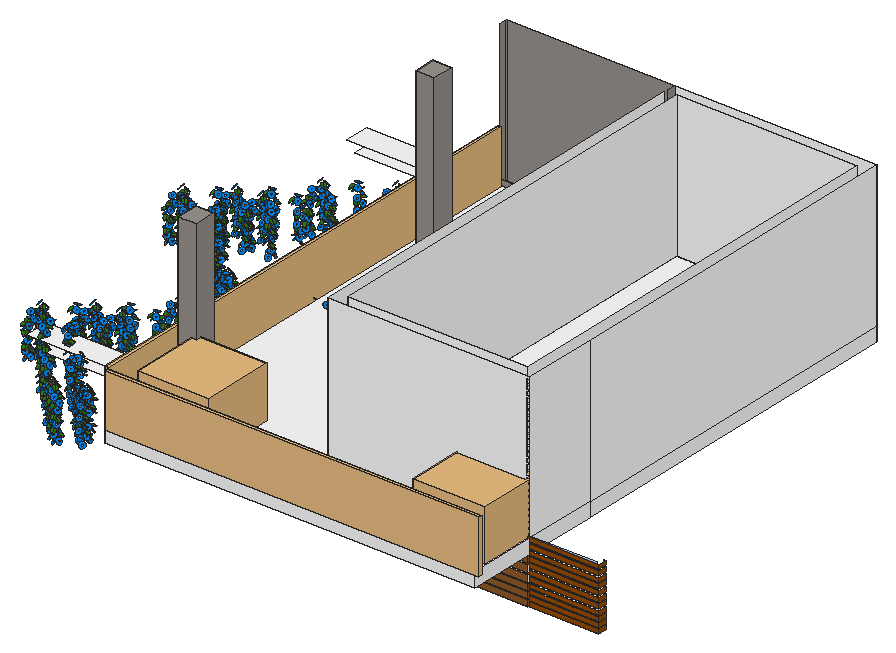
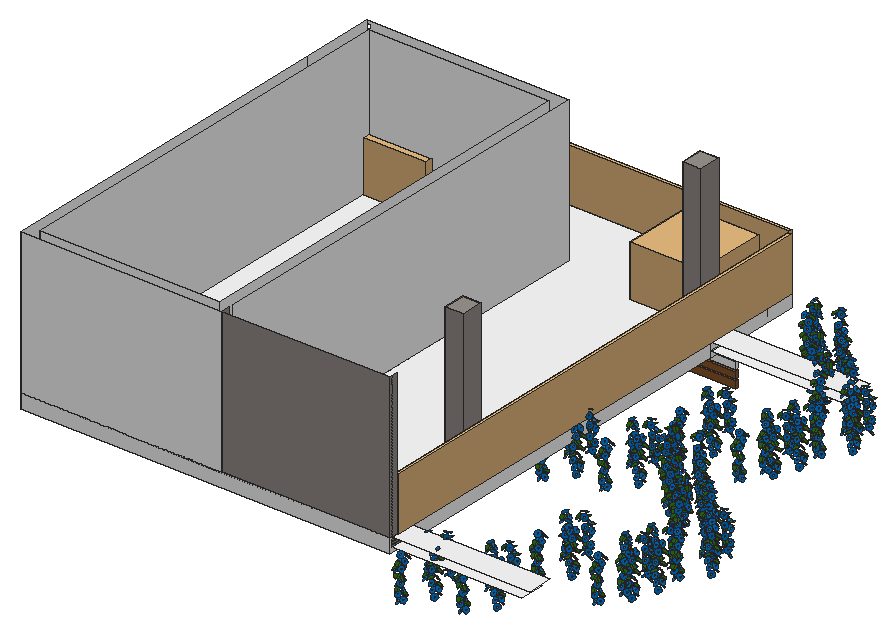
# SketchUp Ruby script. Lengths in inches.
U = 1.inch
M = Sketchup.active_model
def pt(a) = Geom::Point3d.new(a.map { |v| v * U })
def face(e, loops, mat)
  f = e.add_face(loops[0].map { |a| pt(a) })
  loops[1..].each { |l| e.add_face(l.map { |a| pt(a) }).erase! }
  f.material = f.back_material = mat if mat
  f
end
# faces: each face lists its corners as indices into pts; further lists are holes
def faces(e, pts, list, mat = nil) = list.each { |f| face(e, (f[0].is_a?(Array) ? f : [f]).map { |l| l.map { |i| pts[i] } }, mat) }
# xy, xz, yz: faces in a plane at the given z, y or x. An outline is a flat list of corners, or four numbers for a rectangle; further outlines are holes
def ring(l) = l.size == 4 ? [[l[0], l[1]], [l[2], l[1]], [l[2], l[3]], [l[0], l[3]]] : l.each_slice(2).to_a
def flat(e, list, mat, &to3) = list.each { |f| face(e, (f[0].is_a?(Array) ? f : [f]).map { |l| ring(l).map { |u, v| to3.(u, v) } }, mat) }
def xy(e, z, list, mat = nil) = flat(e, list, mat) { |x, y| [x, y, z] }
def xz(e, y, list, mat = nil) = flat(e, list, mat) { |x, z| [x, y, z] }
def yz(e, x, list, mat = nil) = flat(e, list, mat) { |y, z| [x, y, z] }
def lines(e, pts, list) = list.each { |a, b| e.add_line(pt(pts[a]), pt(pts[b])) }
# prism: a flat outline (further loops are holes) pulled along v
def prism(e, loops, v, mat = nil)
  f = face(e, loops, mat); d = Geom::Vector3d.new(v.map { |x| x * U })
  f.pushpull(f.normal.samedirection?(d) ? d.length : -d.length)
end
def box(e, o, s, mat = nil) = prism(e, [[o, [o[0] + s[0], o[1], o[2]], [o[0] + s[0], o[1] + s[1], o[2]], [o[0], o[1] + s[1], o[2]]]], [0, 0, s[2]], mat)
def at(x, y, z, deg = 0) = Geom::Transformation.translation(pt([x, y, z])) * Geom::Transformation.rotation(ORIGIN, Z_AXIS, deg.degrees)
def axes(o, x, y, z) = Geom::Transformation.new([*x, 0, *y, 0, *z, 0, *pt(o).to_a, 1])
def part(name) = M.definitions.add(name)
# library, detail: a bought-in or finely detailed component or shape, given as its bounding box
def library(name, o, s) = part(name).tap { |d| box(d.entities, o, s) }
def detail(e, o, s) = box(e.add_group.entities, o, s)
def put(e, d, t, mat = nil) = e.add_instance(d, t).tap { |i| i.material = mat if mat }
def group(e, t, mat = nil) = e.add_group.tap { |g| g.transformation = t; g.material = mat if mat }.entities
root = M.entities
M.materials.add("[Color C07]").color = [153, 76, 0]
M.materials.add("[Color M00]").color = [255, 255, 255]
M.materials.add("[Granite Tile]").color = [155, 148, 143]
M.materials.add("[Translucent Glass Blue]").color = [100, 149, 237]
M.materials["[Translucent Glass Blue]"].alpha = 0.5
M.materials.add("[Wood Floor Parquet]").color = [145, 89, 39]
M.materials.add("skp avat flo 1").color = [0, 129, 229]
M.materials.add("skp avat flo 2").color = [47, 120, 22]
c1 = part("Gruppe\#2")
xy(c1.entities,0,[[6.69,0,4.96,0.23,3.03,1.59,1.96,1.96,0.9,3.35,0.9,5.71,0,6.69,0.23,8.43,1.96,10,3.35,12.49,4.67,13.04,7.04,12.49,8.72,13.04,10.04,12.49,11.43,11.43,12.05,9.15,13.39,6.69,13.16,4.96,12.49,3.35,10.41,2.22,8.43,0.23]],"skp avat flo 1")
c2 = part("Gruppe\#12")
xy(c2.entities,0,[[1.18,0.5,1.36,0.52,1.52,0.59,1.67,0.7,1.77,0.84,1.84,1,1.87,1.18,1.84,1.36,1.77,1.52,1.67,1.67,1.52,1.77,1.36,1.84,1.18,1.87,1,1.84,0.84,1.77,0.7,1.67,0.59,1.52,0.52,1.36,0.5,1.18,0.52,1,0.59,0.84,0.7,0.7,0.84,0.59,1,0.52]])
c3 = part("f.st. wop plant 01 blüte")
put(c3.entities,c1,at(0,0,0))
put(c3.entities,c2,at(5.65,5.41,0.39))
c4 = part("Gruppe\#5")
xy(c4.entities,0.96,[[13.97,0.22,8.73,4.42,7.37,10.11,8.43,14.53,13.97,16.39]],"skp avat flo 2")
p = [[13.97,0.22,0.96],[13.97,16.39,0.96],[17.89,14.53,4.875],[18.64,10.11,5.625],[17.67,4.42,4.66]]
faces(c4.entities,p,[[0,1,2,3,4]],"skp avat flo 2")
c5 = part("f.st. wop plant 01 blatt")
put(c5.entities,c4,axes([0.99,0,4.74],[0.91566,0,-0.40195],[0,1,0],[0.40195,0,0.91566]))
c6 = part("Gruppe\#10")
put(c6.entities,c3,axes([4.61,0.45,57.14],[0.99373,-0.06775,-0.08889],[0.11172,0.62588,0.77188],[0.00335,-0.77697,0.62953]))
put(c6.entities,c3,axes([12.4,0.4,0.59],[0.70061,0.70799,-0.08889],[-0.40079,0.49353,0.77188],[0.59035,-0.50516,0.62953]))
put(c6.entities,c3,axes([24.4375,6.09,17.58],[-0.05734,0.99439,-0.08889],[-0.63495,0.03239,0.77188],[0.77043,0.1007,0.62953]))
put(c6.entities,c3,axes([1.11,8.09,13.25],[0.88983,-0.44754,-0.08889],[0.34553,0.53368,0.77188],[-0.298,-0.71756,0.62953]))
put(c6.entities,c3,axes([23.26,15,37.53],[-0.84836,0.52191,-0.08889],[-0.38985,-0.50222,0.77188],[0.35821,0.68948,0.62953]))
put(c6.entities,c3,axes([12.67,23.61,24.88],[-0.75852,-0.64555,-0.08889],[0.35717,-0.52596,0.77188],[-0.54504,0.55374,0.62953]))
put(c6.entities,c3,axes([20.43,22.9,81.42],[-0.98432,0.15238,-0.08889],[-0.16477,-0.61405,0.77188],[0.06303,0.77442,0.62953]))
put(c6.entities,c3,axes([1.76,2.9,29.21],[0.93833,-0.33412,-0.08889],[0.27691,0.5723,0.77188],[-0.20703,-0.74889,0.62953]))
put(c6.entities,c3,axes([13.59,0.5,77.09],[0.62412,0.77625,-0.08889],[-0.4494,0.44972,0.77188],[0.63915,-0.4418,0.62953]))
put(c6.entities,c3,axes([-1.26,15.51,69.79],[0.24265,-0.96603,-0.08889],[0.62977,0.08716,0.77188],[-0.73791,-0.24328,0.62953]))
put(c6.entities,c3,axes([22.04,17.92,65.46],[-0.95793,0.27287,-0.08889],[-0.2394,-0.58898,0.77188],[0.15827,0.76069,0.62953]))
put(c6.entities,c3,axes([9.51,23.35,52.81],[-0.55554,-0.82673,-0.08889],[0.48617,-0.40969,0.77188],[-0.67455,0.38559,0.62953]))
put(c6.entities,c3,axes([0.1875,18.97,41.86],[-0.02781,-0.99565,-0.08889],[0.62986,-0.08651,0.77188],[-0.77621,-0.03452,0.62953]))
put(c6.entities,c3,axes([24.98,7.4,94.08],[-0.15925,0.98323,-0.08889],[-0.63491,-0.03305,0.77188],[0.75599,0.17936,0.62953]))
put(c6.entities,c3,axes([21.5,21.98,4.93],[-0.96344,0.25275,-0.08889],[-0.22702,-0.59386,0.77188],[0.1423,0.76384,0.62953]))
put(c6.entities,c3,axes([1.57,6.98,89.75],[0.93112,-0.3537,-0.08889],[0.28884,0.56637,0.77188],[-0.22267,-0.74439,0.62953]))
put(c6.entities,c5,axes([9.37,32.32,90.95],[-0.51317,-0.65235,0],[0.5996,-0.47167,0.32697],[-0.25699,0.20216,0.76288]))
put(c6.entities,c5,axes([33.81,6.72,78.35],[-0.27992,0.78137,0],[-0.71819,-0.25729,0.32697],[0.30782,0.11027,0.76288]))
put(c6.entities,c5,axes([-9.46,14.86,61.47],[0.53029,-0.63851,0],[0.58688,0.4874,0.32697],[-0.25154,-0.2089,0.76288]))
put(c6.entities,c5,axes([21.49,-6.15,66.98],[0.2591,0.78852,0],[-0.72476,0.23815,0.32697],[0.31063,-0.10207,0.76288]))
put(c6.entities,c5,axes([32.03,5.27,54.38],[-0.36397,0.74594,0],[-0.68562,-0.33454,0.32697],[0.29386,0.14338,0.76288]))
put(c6.entities,c5,axes([30.63,20.6,49.31],[-0.77544,0.29596,0],[-0.27203,-0.71273,0.32697],[0.11659,0.30548,0.76288]))
put(c6.entities,c5,axes([32.03,5.27,27.16],[-0.36397,0.74594,0],[-0.68562,-0.33454,0.32697],[0.29386,0.14338,0.76288]))
put(c6.entities,c5,axes([17.4375,27.53,13.8125],[-0.76735,-0.23527,0.21148],[0.29408,-0.735,0.24937],[0.11659,0.30548,0.76288]))
put(c6.entities,c5,axes([-9.46,14.86,34.24],[0.53029,-0.63851,0],[0.58688,0.4874,0.32697],[-0.25154,-0.2089,0.76288]))
c7 = part("Gruppe\#9")
put(c7.entities,c3,axes([2.2,1.62,57.61],[0.97169,-0.0623,-0.22792],[0.22172,0.57378,0.78843],[0.08166,-0.81664,0.57134]))
put(c7.entities,c3,axes([-1.48,7.53,1.27],[0.68093,0.71536,-0.15682],[-0.22028,0.40428,0.88771],[0.69843,-0.56993,0.43287]))
put(c7.entities,c3,axes([13.97,11.34,15.86],[-0.0542,0.99797,0.03349],[-0.45869,-0.05467,0.88691],[0.88694,0.03271,0.46072]))
put(c7.entities,c3,axes([-9.71,13.74,16.77],[0.84218,-0.4326,-0.32186],[0.5102,0.4462,0.73526],[-0.17446,-0.78343,0.59649]))
put(c7.entities,c3,axes([17.17,17.99,36.46],[-0.83727,0.52624,0.14846],[-0.23006,-0.58536,0.77745],[0.49603,0.61679,0.61117]))
put(c7.entities,c3,axes([4.35,27.92,27.32],[-0.77345,-0.63385,0.00301],[0.4998,-0.60694,0.61792],[-0.38984,0.47943,0.78623]))
put(c7.entities,c3,axes([20.43,22.9,81.42],[-0.98432,0.15238,-0.08889],[-0.16477,-0.61405,0.77188],[0.06303,0.77442,0.62953]))
put(c7.entities,c3,axes([-5.84,6.82,31.58],[0.89192,-0.31974,-0.31975],[0.44391,0.4844,0.75386],[-0.08616,-0.81432,0.57398]))
put(c7.entities,c3,axes([13.59,0.5,77.09],[0.62412,0.77625,-0.08889],[-0.4494,0.44972,0.77188],[0.63915,-0.4418,0.62953]))
put(c7.entities,c3,axes([-1.26,15.51,69.79],[0.24265,-0.96603,-0.08889],[0.62977,0.08716,0.77188],[-0.73791,-0.24328,0.62953]))
put(c7.entities,c3,axes([20.77,18.5,64.59],[-0.95848,0.27864,0.06062],[-0.13765,-0.63827,0.75741],[0.24973,0.71762,0.65012]))
put(c7.entities,c3,axes([6.6875,24.75,54.15],[-0.57029,-0.8188,-0.06577],[0.58283,-0.45976,0.67002],[-0.57885,0.34377,0.73942]))
put(c7.entities,c3,axes([-4.08,21.11,44.3125],[-0.04911,-0.98765,-0.14878],[0.72825,-0.13735,0.67141],[-0.68355,-0.07538,0.726]))
put(c7.entities,c3,axes([24.98,7.4,94.08],[-0.15925,0.98323,-0.08889],[-0.63491,-0.03305,0.77188],[0.75599,0.17936,0.62953]))
put(c7.entities,c3,axes([8.77,28.52,5.9],[-0.95532,0.25842,0.14346],[-0.07274,-0.676,0.7333],[0.28648,0.6901,0.6646]))
put(c7.entities,c3,axes([1.57,6.98,89.75],[0.93112,-0.3537,-0.08889],[0.28884,0.56637,0.77188],[-0.22267,-0.74439,0.62953]))
put(c7.entities,c5,axes([9.37,32.32,90.95],[-0.51317,-0.65235,0],[0.5996,-0.47167,0.32697],[-0.25699,0.20216,0.76288]))
put(c7.entities,c5,axes([33.81,6.72,78.35],[-0.27992,0.78137,0],[-0.71819,-0.25729,0.32697],[0.30782,0.11027,0.76288]))
put(c7.entities,c5,axes([-11.01,15.72,64.74],[0.51926,-0.63742,-0.11388],[0.63054,0.46456,0.27478],[-0.14729,-0.25842,0.77487]))
put(c7.entities,c5,axes([20.21,-5.625,64.6],[0.26417,0.78668,0.01588],[-0.67119,0.21655,0.43762],[0.41063,-0.15212,0.70508]))
put(c7.entities,c5,axes([29.04,6.59,51.45],[-0.35348,0.74452,0.09816],[-0.63785,-0.35493,0.39506],[0.39635,0.09281,0.72332]))
put(c7.entities,c5,axes([27.11,22.23,47.625],[-0.76537,0.29574,0.12508],[-0.23173,-0.73252,0.31403],[0.22228,0.25465,0.75805]))
put(c7.entities,c5,axes([23.375,9.49,23.48],[-0.34051,0.7404,0.15735],[-0.60881,-0.37042,0.42548],[0.44978,0.05914,0.69506]))
put(c7.entities,c5,axes([6.77,33.04,15.99],[-0.71083,-0.25923,0.3412],[0.32455,-0.75723,0.10082],[0.2798,0.21977,0.74988]))
put(c7.entities,c5,axes([-15.51,18.125,40.12],[0.50532,-0.63318,-0.18065],[0.65217,0.44994,0.24724],[-0.09068,-0.29247,0.77145]))
c8 = part("Gruppe\#11")
put(c8.entities,c3,axes([4.61,0.45,57.14],[0.99373,-0.06775,-0.08889],[0.11172,0.62588,0.77188],[0.00335,-0.77697,0.62953]))
put(c8.entities,c3,axes([12.4,0.4,0.59],[0.70061,0.70799,-0.08889],[-0.40079,0.49353,0.77188],[0.59035,-0.50516,0.62953]))
put(c8.entities,c3,axes([24.4375,6.09,17.58],[-0.05734,0.99439,-0.08889],[-0.63495,0.03239,0.77188],[0.77043,0.1007,0.62953]))
put(c8.entities,c3,axes([1.11,8.09,13.25],[0.88983,-0.44754,-0.08889],[0.34553,0.53368,0.77188],[-0.298,-0.71756,0.62953]))
put(c8.entities,c3,axes([23.26,15,37.53],[-0.84836,0.52191,-0.08889],[-0.38985,-0.50222,0.77188],[0.35821,0.68948,0.62953]))
put(c8.entities,c3,axes([12.67,23.61,24.88],[-0.75852,-0.64555,-0.08889],[0.35717,-0.52596,0.77188],[-0.54504,0.55374,0.62953]))
put(c8.entities,c3,axes([20.43,22.9,81.42],[-0.98432,0.15238,-0.08889],[-0.16477,-0.61405,0.77188],[0.06303,0.77442,0.62953]))
put(c8.entities,c3,axes([1.76,2.9,29.21],[0.93833,-0.33412,-0.08889],[0.27691,0.5723,0.77188],[-0.20703,-0.74889,0.62953]))
put(c8.entities,c3,axes([13.59,0.5,77.09],[0.62412,0.77625,-0.08889],[-0.4494,0.44972,0.77188],[0.63915,-0.4418,0.62953]))
put(c8.entities,c3,axes([-1.26,15.51,69.79],[0.24265,-0.96603,-0.08889],[0.62977,0.08716,0.77188],[-0.73791,-0.24328,0.62953]))
put(c8.entities,c3,axes([22.04,17.92,65.46],[-0.95793,0.27287,-0.08889],[-0.2394,-0.58898,0.77188],[0.15827,0.76069,0.62953]))
put(c8.entities,c3,axes([9.51,23.35,52.81],[-0.55554,-0.82673,-0.08889],[0.48617,-0.40969,0.77188],[-0.67455,0.38559,0.62953]))
put(c8.entities,c3,axes([0.1875,18.97,41.86],[-0.02781,-0.99565,-0.08889],[0.62986,-0.08651,0.77188],[-0.77621,-0.03452,0.62953]))
put(c8.entities,c3,axes([24.98,7.4,94.08],[-0.15925,0.98323,-0.08889],[-0.63491,-0.03305,0.77188],[0.75599,0.17936,0.62953]))
put(c8.entities,c3,axes([21.5,21.98,4.93],[-0.96344,0.25275,-0.08889],[-0.22702,-0.59386,0.77188],[0.1423,0.76384,0.62953]))
put(c8.entities,c3,axes([1.57,6.98,89.75],[0.93112,-0.3537,-0.08889],[0.28884,0.56637,0.77188],[-0.22267,-0.74439,0.62953]))
put(c8.entities,c5,axes([9.37,32.32,90.95],[-0.51317,-0.65235,0],[0.5996,-0.47167,0.32697],[-0.25699,0.20216,0.76288]))
put(c8.entities,c5,axes([33.81,6.72,78.35],[-0.27992,0.78137,0],[-0.71819,-0.25729,0.32697],[0.30782,0.11027,0.76288]))
put(c8.entities,c5,axes([-9.46,14.86,61.47],[0.53029,-0.63851,0],[0.58688,0.4874,0.32697],[-0.25154,-0.2089,0.76288]))
put(c8.entities,c5,axes([21.49,-6.15,66.98],[0.2591,0.78852,0],[-0.72476,0.23815,0.32697],[0.31063,-0.10207,0.76288]))
put(c8.entities,c5,axes([32.03,5.27,54.38],[-0.36397,0.74594,0],[-0.68562,-0.33454,0.32697],[0.29386,0.14338,0.76288]))
put(c8.entities,c5,axes([30.63,20.6,49.31],[-0.77544,0.29596,0],[-0.27203,-0.71273,0.32697],[0.11659,0.30548,0.76288]))
put(c8.entities,c5,axes([32.03,5.27,27.16],[-0.36397,0.74594,0],[-0.68562,-0.33454,0.32697],[0.29386,0.14338,0.76288]))
put(c8.entities,c5,axes([17.4375,27.53,13.8125],[-0.76735,-0.23527,0.21148],[0.29408,-0.735,0.24937],[0.11659,0.30548,0.76288]))
put(c8.entities,c5,axes([-9.46,14.86,34.24],[0.53029,-0.63851,0],[0.58688,0.4874,0.32697],[-0.25154,-0.2089,0.76288]))
c9 = part("Gruppe\#8")
put(c9.entities,c3,axes([2.26,1.13,59.39],[0.92531,-0.05375,-0.37538],[0.3384,0.56379,0.75341],[0.17114,-0.82417,0.53987]))
put(c9.entities,c3,axes([-9.39,6.25,4.33],[0.64151,0.72107,-0.26176],[-0.09814,0.41557,0.90425],[0.76081,-0.5544,0.33735]))
put(c9.entities,c3,axes([7.9,10.48,16.53],[-0.06325,0.99763,0.02691],[-0.32763,-0.04623,0.94367],[0.94269,0.05087,0.32978]))
put(c9.entities,c3,axes([-15.4375,12.6,20.76],[0.79424,-0.42729,-0.43198],[0.60271,0.46401,0.64918],[-0.07695,-0.77596,0.62607]))
put(c9.entities,c3,axes([13.9,17.49,36.37],[-0.81529,0.51823,0.25834],[-0.1092,-0.57574,0.81031],[0.56867,0.63242,0.52599]))
put(c9.entities,c3,axes([-0.23,27.12,29.01],[-0.75604,-0.64315,0.1215],[0.59094,-0.59091,0.5492],[-0.28142,0.48702,0.82681]))
put(c9.entities,c3,axes([20.43,22.9,81.42],[-0.98432,0.15238,-0.08889],[-0.16477,-0.61405,0.77188],[0.06303,0.77442,0.62953]))
put(c9.entities,c3,axes([-9.41,5.97,34.96],[0.84215,-0.31382,-0.43852],[0.53918,0.50168,0.67646],[0.00771,-0.80612,0.5917]))
put(c9.entities,c3,axes([13.59,0.5,77.09],[0.62412,0.77625,-0.08889],[-0.4494,0.44972,0.77188],[0.63915,-0.4418,0.62953]))
put(c9.entities,c3,axes([-1.26,15.51,69.79],[0.24265,-0.96603,-0.08889],[0.62977,0.08716,0.77188],[-0.73791,-0.24328,0.62953]))
put(c9.entities,c3,axes([22.04,17.92,65.46],[-0.95793,0.27287,-0.08889],[-0.2394,-0.58898,0.77188],[0.15827,0.76069,0.62953]))
put(c9.entities,c3,axes([6.08,24.33,55.62],[-0.57097,-0.82091,0.01051],[0.68037,-0.46598,0.56565],[-0.45945,0.33012,0.82458]))
put(c9.entities,c3,axes([-6.06,20.77,47.51],[-0.06819,-0.9857,-0.15407],[0.82323,-0.14283,0.54945],[-0.56361,-0.08937,0.8212]))
put(c9.entities,c3,axes([24.98,7.4,94.08],[-0.15925,0.98323,-0.08889],[-0.63491,-0.03305,0.77188],[0.75599,0.17936,0.62953]))
put(c9.entities,c3,axes([1.11,27.4375,7.17],[-0.92899,0.24893,0.27387],[0.04156,-0.66514,0.74556],[0.36776,0.70401,0.60756]))
put(c9.entities,c3,axes([1.57,6.98,89.75],[0.93112,-0.3537,-0.08889],[0.28884,0.56637,0.77188],[-0.22267,-0.74439,0.62953]))
put(c9.entities,c5,axes([9.37,32.32,90.95],[-0.51317,-0.65235,0],[0.5996,-0.47167,0.32697],[-0.25699,0.20216,0.76288]))
put(c9.entities,c5,axes([33.81,6.72,78.35],[-0.27992,0.78137,0],[-0.71819,-0.25729,0.32697],[0.30782,0.11027,0.76288]))
put(c9.entities,c5,axes([-9.74,15.05,68.68],[0.49765,-0.63289,-0.20172],[0.66377,0.46408,0.1815],[-0.02561,-0.27014,0.78439]))
put(c9.entities,c5,axes([21.49,-6.15,66.98],[0.2591,0.78852,0],[-0.72476,0.23815,0.32697],[0.31063,-0.10207,0.76288]))
put(c9.entities,c5,axes([27.8125,6.34,49.26],[-0.33661,0.74111,0.1623],[-0.5684,-0.36396,0.48306],[0.5025,0.08476,0.65514]))
put(c9.entities,c5,axes([25.26,22.01,46],[-0.73801,0.28975,0.24554],[-0.17833,-0.73814,0.33502],[0.33532,0.24514,0.71859]))
put(c9.entities,c5,axes([18.32,8.86,22.77],[-0.32541,0.73857,0.19371],[-0.53703,-0.37106,0.51265],[0.54278,0.07565,0.62335]))
put(c9.entities,c5,axes([0.49,32.09,17.38],[-0.65154,-0.26248,0.44214],[0.34641,-0.75151,0.06433],[0.37999,0.23503,0.69948]))
put(c9.entities,c5,axes([-17.94,17.29,44.63],[0.48369,-0.62973,-0.24163],[0.67408,0.46176,0.14595],[0.0237,-0.2813,0.78052]))
c10 = part("f.st. wop plant 01")
put(c10.entities,c6,at(39.14,64.09,18.66,-141.2))
put(c10.entities,c7,axes([53.54,120.93,12.24],[-0.61849,0.75929,0.20233],[-0.78178,-0.62056,-0.06099],[0.07925,-0.1959,0.97742]))
put(c10.entities,c8,at(82.26,36.89,18.66))
put(c10.entities,c9,axes([72.55,-5.87,29.3],[0.62579,-0.70508,0.33355],[0.76326,0.64164,-0.07566],[-0.16067,0.30193,0.93969]))
c11 = part("World of Pandora - tree 01")
put(c11.entities,c10,at(57.06,8.63,0))
c12 = part("Group\#17")
box(c12.entities,[0,-2.125,0],[58.6875,4.9375,2.3125])
c13 = library("CM1021-ceilingfixture-VisaLighting.dwg",[51.34,51.34,0],[17.32,17.32,4.91])
c14 = part("CM1021")
put(c14.entities,c13,at(-75.2,7.58,71.26,-15))
put(c14.entities,c13,at(67.3,7.58,71.26,-15))
put(c14.entities,c13,at(180.18,7.58,71.26,-15))
c15 = library("Skt_BoxwoodBall_13",[-7.4,-7.46,-2.06],[14.58,14.83,12.98])
c16 = library("Glass railing panel",[0.75,0.33,0],[60,3.22,44.35])
c17 = part("Group\#30")
box(c17.entities,[0,0,0],[15.375,18.4375,128.42])
xy(root,213.84,[[561.375,211.8125,561.375,213.625,622.25,213.625,622.25,218.625,623.5625,218.625,623.5625,211.8125]],"[Color M00]")
xy(root,217.4,[[561.375,211.8125,623.5625,211.8125,623.5625,218.625,622.25,218.625,622.25,213.625,561.375,213.625]],"[Color M00]")
xy(root,218.15,[[561.375,211.8125,561.375,213.625,622.25,213.625,622.25,218.625,623.5625,218.625,623.5625,211.8125]],"[Color M00]")
xy(root,221.71,[[561.375,211.8125,623.5625,211.8125,623.5625,218.625,622.25,218.625,622.25,213.625,561.375,213.625]],"[Color M00]")
xy(root,222.96,[[561.375,211.8125,561.375,213.625,622.25,213.625,622.25,218.625,623.5625,218.625,623.5625,211.8125]],"[Color M00]")
xy(root,226.52,[[561.375,211.8125,623.5625,211.8125,623.5625,218.625,622.25,218.625,622.25,213.625,561.375,213.625]],"[Color M00]")
xy(root,227.46,[[561.375,211.8125,561.375,213.625,622.25,213.625,622.25,218.625,623.5625,218.625,623.5625,211.8125]],"[Color M00]")
xy(root,231.02,[[561.375,211.8125,623.5625,211.8125,623.5625,218.625,622.25,218.625,622.25,213.625,561.375,213.625]],"[Color M00]")
xy(root,232.46,[[561.375,211.8125,561.375,213.625,622.25,213.625,622.25,218.625,623.5625,218.625,623.5625,211.8125]],"[Color M00]")
xy(root,236.02,[[561.375,211.8125,623.5625,211.8125,623.5625,218.625,622.25,218.625,622.25,213.625,561.375,213.625]],"[Color M00]")
xy(root,237.27,[[561.375,211.8125,561.375,213.625,622.25,213.625,622.25,218.625,623.5625,218.625,623.5625,211.8125]],"[Color M00]")
xy(root,240.84,[[561.375,211.8125,623.5625,211.8125,623.5625,218.625,622.25,218.625,622.25,213.625,561.375,213.625]],"[Color M00]")
xy(root,242.46,[[561.375,211.8125,561.375,213.625,622.25,213.625,622.25,218.625,623.5625,218.625,623.5625,211.8125]],"[Color M00]")
xy(root,246.02,[[561.375,211.8125,623.5625,211.8125,623.5625,218.625,622.25,218.625,622.25,213.625,561.375,213.625]],"[Color M00]")
xy(root,247.4,[[561.375,211.8125,561.375,213.625,622.25,213.625,622.25,218.625,623.5625,218.625,623.5625,211.8125]],"[Color M00]")
xy(root,250.96,[[561.375,211.8125,623.5625,211.8125,623.5625,218.625,622.25,218.625,622.25,213.625,561.375,213.625]],"[Color M00]")
xy(root,252,[[[257.3125,213.625,564.8125,573.625],[266.75,222.625,555.8125,564.625]]],"[Color M00]")
xy(root,252.09,[[561.375,211.8125,561.375,213.625,622.25,213.625,622.25,218.625,623.5625,218.625,623.5625,211.8125]],"[Color M00]")
xy(root,255.65,[[561.375,211.8125,623.5625,211.8125,623.5625,218.625,622.25,218.625,622.25,213.625,561.375,213.625]],"[Color M00]")
xy(root,256.75,[[149.03,219.03,257.3125,239.92],[149.03,551.125,257.3125,572.01]],"[Color M00]")
xy(root,257.02,[[561.375,211.8125,561.375,213.625,622.25,213.625,622.25,218.625,623.5625,218.625,623.5625,211.8125]],"[Color M00]")
xy(root,260.59,[[561.375,211.8125,623.5625,211.8125,623.5625,218.625,622.25,218.625,622.25,213.625,561.375,213.625]],"[Color M00]")
xy(root,262.02,[[561.375,211.8125,561.375,213.625,622.25,213.625,622.25,218.625,623.5625,218.625,623.5625,211.8125]],"[Color M00]")
xy(root,264,[[[396.75,213.625,564.8125,573.625],[405.75,222.625,555.8125,564.625]],[141.8125,219.03,257.3125,239.92],[405.75,222.625,555.8125,564.625],[141.8125,551.125,257.3125,572.01]],"[Color M00]")
xy(root,264,[[257.3125,566.64,396.75,573.625]],"[Granite Tile]")
xz(root,211.8125,[[561.375,213.84,623.5625,217.4],[561.375,218.15,623.5625,221.71],[561.375,222.96,623.5625,226.52],[561.375,227.46,623.5625,231.02],[561.375,232.46,623.5625,236.02],
  [561.375,237.27,623.5625,240.84],[561.375,242.46,623.5625,246.02],[561.375,247.4,623.5625,250.96],[561.375,252.09,623.5625,255.65],[561.375,257.02,623.5625,260.59],
  [561.375,262.02,623.5625,265.59]],"[Color C07]")
xz(root,213.625,[[561.375,213.84,564.8125,217.4],[561.375,218.15,564.8125,221.71],[561.375,222.96,564.8125,226.52],[561.375,227.46,564.8125,231.02],[561.375,232.46,564.8125,236.02],
  [561.375,237.27,564.8125,240.84],[561.375,242.46,564.8125,246.02],[396.75,264,561.375,264,561.375,265.59,564.8125,265.59,564.8125,266.65,561.375,266.65,561.375,270.21,564.8125,270.21,564.8125,271.27,561.375,271.27,561.375,274.84,564.8125,274.84,564.8125,276.02,561.375,276.02,561.375,279.59,564.8125,279.59,564.8125,280.85,561.375,280.85,561.375,284.41,564.8125,284.41,564.8125,285.72,561.375,285.72,561.375,289.29,564.8125,289.29,564.8125,290.1,561.375,290.1,561.375,293.66,564.8125,293.66,564.8125,294.97,561.375,294.97,561.375,298.54,564.8125,298.54,564.8125,299.91,561.375,299.91,561.375,303.47,564.8125,303.47,564.8125,304.72,561.375,304.72,561.375,308.29,564.8125,308.29,564.8125,309.6,561.375,309.6,561.375,313.16,564.8125,313.16,564.8125,314.54,561.375,314.54,561.375,318.1,564.8125,318.1,564.8125,319.1,561.375,319.1,561.375,322.66,564.8125,322.66,564.8125,323.85,561.375,323.85,561.375,327.41,564.8125,327.41,564.8125,328.35,561.375,328.35,561.375,331.91,564.8125,331.91,564.8125,333.1,561.375,333.1,561.375,336.66,564.8125,336.66,564.8125,337.48,561.375,337.48,561.375,341.04,564.8125,341.04,564.8125,342.04,561.375,342.04,561.375,345.6,564.8125,345.6,564.8125,346.54,561.375,346.54,561.375,350.1,564.8125,350.1,564.8125,350.85,561.375,350.85,561.375,354.41,564.8125,354.41,564.8125,355.35,561.375,355.35,561.375,358.91,564.8125,358.91,564.8125,359.73,561.375,359.73,561.375,363.29,564.8125,363.29,564.8125,364.29,561.375,364.29,561.375,367.85,564.8125,367.85,564.8125,368.98,561.375,368.98,561.375,372.54,564.8125,372.54,564.8125,373.79,561.375,373.79,561.375,377.35,564.8125,377.35,564.8125,378.41,561.375,378.41,561.375,381.98,564.8125,381.98,564.8125,384,396.75,384],[561.375,264,564.8125,265.59]],"[Color M00]")
xz(root,213.625,[[564.8125,213.84,620.9375,217.4],[564.8125,217.4,620.9375,218.15],[564.8125,218.15,620.9375,221.71],[564.8125,221.71,620.9375,222.96],[564.8125,222.96,620.9375,226.52],
  [564.8125,226.52,620.9375,227.46],[564.8125,227.46,620.9375,231.02],[564.8125,231.02,620.9375,232.46],[564.8125,232.46,620.9375,236.02],[564.8125,236.02,620.9375,237.27],
  [564.8125,237.27,620.9375,240.84],[564.8125,240.84,620.9375,242.46],[564.8125,242.46,620.9375,246.02],[564.8125,246.02,620.9375,247.4],[564.8125,247.4,620.9375,250.96],
  [564.8125,250.96,620.9375,252.09],[564.8125,252.09,620.9375,255.65],[564.8125,255.65,620.9375,257.02],[564.8125,257.02,620.9375,260.59],[564.8125,260.59,620.9375,262.02],
  [564.8125,262.02,620.9375,265.59]],"[Translucent Glass Blue]")
xz(root,218.625,[[622.25,213.84,623.5625,217.4],[622.25,218.15,623.5625,221.71],[622.25,222.96,623.5625,226.52],[622.25,227.46,623.5625,231.02],[622.25,232.46,623.5625,236.02],
  [622.25,237.27,623.5625,240.84],[622.25,242.46,623.5625,246.02],[622.25,247.4,623.5625,250.96],[622.25,252.09,623.5625,255.65],[622.25,257.02,623.5625,260.59],
  [622.25,262.02,623.5625,265.59]],"[Color M00]")
xz(root,222.625,[[405.75,264,555.8125,384]],"[Color M00]")
xz(root,564.625,[[405.75,264,555.8125,384]],"[Color M00]")
xz(root,566.64,[[257.3125,264,396.75,268.5625]],"[Granite Tile]")
xz(root,573.625,[[396.75,264,564.8125,384]],"[Color M00]")
xz(root,573.625,[[257.3125,264,396.75,384]],"[Granite Tile]")
yz(root,257.3125,[[219.03,252,239.92,256.75],[219.03,256.75,239.92,264]],"[Color M00]")
yz(root,257.3125,[[551.125,256.75,572.01,264],[566.64,264,572.01,384],[572.01,264,573.625,384]],"[Granite Tile]")
yz(root,396.75,[[213.625,264,213.625,384,562.2,384,562.2,375.25,566.64,375.25,566.64,287.25,562.2,287.25,562.2,278.5,566.64,278.5,566.64,264]],"[Color M00]")
yz(root,396.75,[[566.64,264,573.625,384]],"[Granite Tile]")
yz(root,405.75,[[222.625,264,564.625,384]],"[Color M00]")
yz(root,555.8125,[[222.625,264,564.625,384]],"[Color M00]")
yz(root,561.375,[[211.8125,213.84,213.625,217.4],[211.8125,218.15,213.625,221.71],[211.8125,222.96,213.625,226.52],[211.8125,227.46,213.625,231.02],[211.8125,232.46,213.625,236.02],
  [211.8125,237.27,213.625,240.84],[211.8125,242.46,213.625,246.02],[211.8125,247.4,213.625,250.96],[211.8125,252.09,213.625,255.65],[211.8125,257.02,213.625,260.59],
  [211.8125,262.02,213.625,265.59]],"[Color M00]")
yz(root,564.8125,[[213.625,252,275.23,264],[213.625,264,275.23,384],[275.23,264,573.625,384]],"[Color M00]")
yz(root,623.5625,[[211.8125,213.84,218.625,217.4],[211.8125,218.15,218.625,221.71],[211.8125,222.96,218.625,226.52],[211.8125,227.46,218.625,231.02],[211.8125,232.46,218.625,236.02],
  [211.8125,237.27,218.625,240.84],[211.8125,242.46,218.625,246.02],[211.8125,247.4,218.625,250.96],[211.8125,252.09,218.625,255.65],[211.8125,257.02,218.625,260.59],
  [211.8125,262.02,218.625,265.59]],"[Color C07]")
p = [[257.3125,180.8125,259.26],[257.3125,180.8125,256.75],[257.3125,180.8125,264]]
lines(root,p,[[0,1],[2,0]])
put(root,c11,axes([95.28,483.59,210.81],[0.26912,-0.25392,0],[0.25392,0.26912,0],[0,0,0.37]),"[Granite Tile]")
put(root,c11,axes([155.87,547.81,211.19],[0.26912,-0.25392,0],[0.25392,0.26912,0],[0,0,0.37]),"[Granite Tile]")
put(root,c12,axes([506.125,213.625,216.02],[1,0,0],[0,0,1],[0,-1,0]),"[Wood Floor Parquet]")
put(root,c11,axes([122.33,302.64,213.44],[0.26912,-0.25392,0],[0.25392,0.26912,0],[0,0,0.37]),"[Granite Tile]")
put(root,c11,axes([159.78,320.09,213.73],[0.25392,0.26912,0],[-0.26912,0.25392,0],[0,0,0.37]),"[Granite Tile]")
put(root,c11,axes([182.92,366.86,213.83],[0.26912,-0.25392,0],[0.25392,0.26912,0],[0,0,0.37]),"[Granite Tile]")
g1 = group(root,at(257.3125,213.625,217.22),"[Color M00]")
box(g1,[0,-2.3125,0],[173.47,2.3125,5.79],"[Wood Floor Parquet]")
put(root,c11,axes([186.83,139.14,216.37],[0.25392,0.26912,0],[-0.26912,0.25392,0],[0,0,0.37]),"[Granite Tile]")
put(root,c11,axes([82.49,472.125,216.49],[0.26912,-0.25392,0],[0.25392,0.26912,0],[0,0,0.37]),"[Granite Tile]")
put(root,c12,axes([506.125,213.625,221.7],[1,0,0],[0,0,1],[0,-1,0]),"[Wood Floor Parquet]")
put(root,c11,axes([134.64,344.76,218.2],[0.25392,0.26912,0],[-0.26912,0.25392,0],[0,0,0.37]),"[Granite Tile]")
put(root,c11,axes([109.55,291.18,219.13],[0.26912,-0.25392,0],[0.25392,0.26912,0],[0,0,0.37]),"[Granite Tile]")
put(root,c11,axes([186.13,575.04,219.84],[0.26912,-0.25392,0],[0.25392,0.26912,0],[0,0,0.37]),"[Granite Tile]")
put(root,c11,axes([161.69,163.81,220.83],[0.25392,0.26912,0],[-0.26912,0.25392,0],[0,0,0.37]),"[Granite Tile]")
g2 = group(root,at(257.3125,213.625,224.41),"[Color M00]")
box(g2,[0,-2.3125,0],[173.47,2.3125,5.79],"[Wood Floor Parquet]")
put(root,c11,axes([61.98,442.47,222.32],[0.26912,-0.25392,0],[0.25392,0.26912,0],[0,0,0.37]),"[Granite Tile]")
put(root,c11,axes([213.1875,394.1,222.47],[0.26912,-0.25392,0],[0.25392,0.26912,0],[0,0,0.37]),"[Granite Tile]")
put(root,c11,axes([175.42,303.82,222.67],[0.25392,0.26912,0],[-0.26912,0.25392,0],[0,0,0.37]),"[Granite Tile]")
put(root,c12,axes([506.125,213.625,227.64],[1,0,0],[0,0,1],[0,-1,0]),"[Wood Floor Parquet]")
put(root,c11,axes([129.13,503.5625,223.91],[0.26912,-0.25392,0],[0.25392,0.26912,0],[0,0,0.37]),"[Granite Tile]")
put(root,c11,axes([89.04,261.52,224.95],[0.26912,-0.25392,0],[0.25392,0.26912,0],[0,0,0.37]),"[Granite Tile]")
put(root,c11,axes([202.47,122.87,225.31],[0.25392,0.26912,0],[-0.26912,0.25392,0],[0,0,0.37]),"[Granite Tile]")
put(root,c11,axes([156.18,322.62,226.54],[0.26912,-0.25392,0],[0.25392,0.26912,0],[0,0,0.37]),"[Granite Tile]")
put(root,c11,axes([115.84,365.61,227.03],[0.25392,0.26912,0],[-0.26912,0.25392,0],[0,0,0.37]),"[Granite Tile]")
g3 = group(root,at(257.3125,213.625,231.58),"[Color M00]")
xy(g3,0,[[0,-2.3125,307.5,0]])
xy(g3,5.79,[[0,-2.3125,307.5,0]])
xz(g3,-2.3125,[[0,0,307.5,5.79]],"[Wood Floor Parquet]")
xz(g3,0,[[0,0,307.5,5.79]])
yz(g3,0,[[-2.3125,0,0,5.79]])
yz(g3,307.5,[[-2.3125,0,0,5.79]])
put(root,c11,axes([142.89,184.66,229.66],[0.25392,0.26912,0],[-0.26912,0.25392,0],[0,0,0.37]),"[Granite Tile]")
g4 = group(root,at(257.3125,213.625,238.9),"[Color M00]")
xy(g4,0,[[0,-2.3125,307.5,0]])
xy(g4,5.79,[[0,-2.3125,307.5,0]])
xz(g4,-2.3125,[[0,0,307.5,5.79]],"[Wood Floor Parquet]")
xz(g4,0,[[0,0,307.5,5.79]])
yz(g4,0,[[-2.3125,0,0,5.79]])
yz(g4,307.5,[[-2.3125,0,0,5.79]])
g5 = group(root,at(257.3125,213.625,246.21),"[Color M00]")
box(g5,[0,-2.3125,0],[307.5,2.3125,5.79],"[Wood Floor Parquet]")
put(root,c14,at(281.23,153.6875,177.125),"[Granite Tile]")
g6 = group(root,at(257.3125,573.625,252),"[Color M00]")
box(g6,[0,-418.125,0],[307.5,418.125,12])
put(root,c15,axes([304.46,198.61,261.74],[4.08,0,0],[0,4.08,0],[0,0,4.08]),"[Granite Tile]")
put(root,c15,axes([533.77,198.61,261.74],[4.08,0,0],[0,4.08,0],[0,0,4.08]),"[Granite Tile]")
put(root,c16,axes([255.76,151.95,264],[5.18774,0,0],[0,1,0],[0,0,1]),"[Color M00]")
put(root,c16,axes([255.81,570.4,264],[0,-6.80265,0],[1,0,0],[0,0,1]),"[Color M00]")
put(root,c17,at(262.72,224.88,264),"[Granite Tile]")
put(root,c17,at(262.72,471.82,264),"[Granite Tile]")
